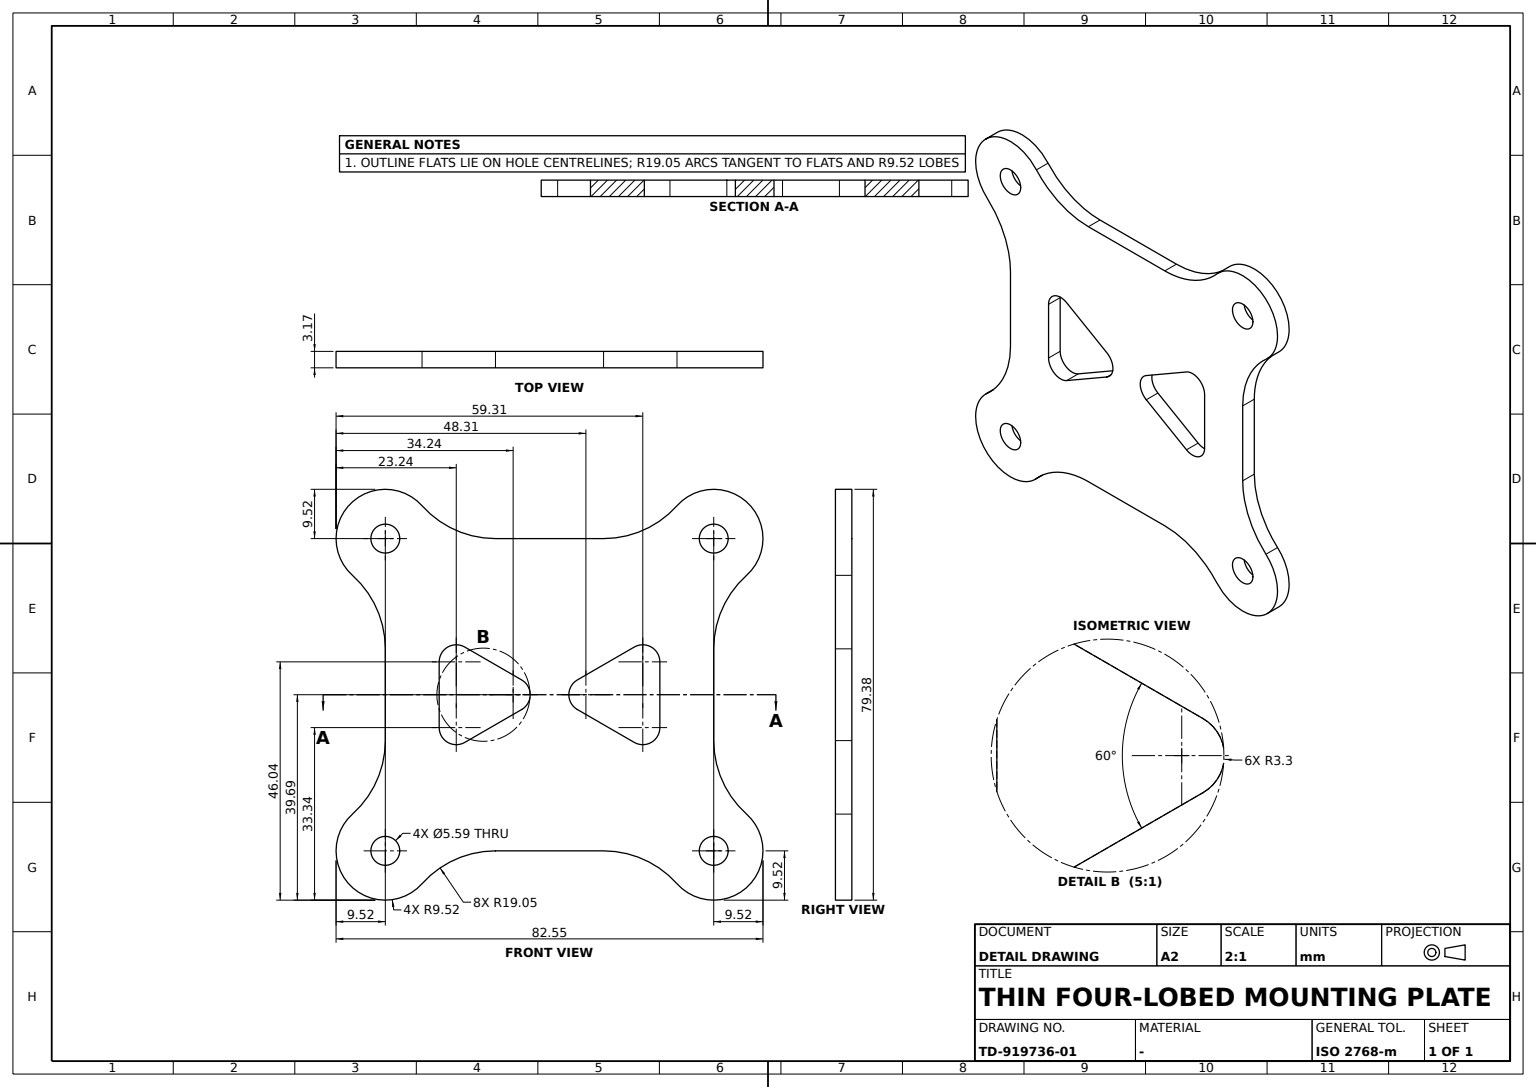
ISO-10303-21;
HEADER;
FILE_DESCRIPTION((''),'2;1');
FILE_NAME('','',(''),(''),'','','');
FILE_SCHEMA(('AUTOMOTIVE_DESIGN'));
ENDSEC;
DATA;
#1=APPLICATION_CONTEXT('');
#2=PRODUCT_CONTEXT('',#1,'mechanical');
#3=PRODUCT('','','',(#2));
#4=PRODUCT_DEFINITION_FORMATION('','',#3);
#5=PRODUCT_DEFINITION_CONTEXT('',#1,'design');
#6=PRODUCT_DEFINITION('','',#4,#5);
#7=PRODUCT_DEFINITION_SHAPE('','',#6);
#8=(LENGTH_UNIT()NAMED_UNIT(*)SI_UNIT(.MILLI.,.METRE.));
#9=(NAMED_UNIT(*)PLANE_ANGLE_UNIT()SI_UNIT($,.RADIAN.));
#10=(NAMED_UNIT(*)SI_UNIT($,.STERADIAN.)SOLID_ANGLE_UNIT());
#11=UNCERTAINTY_MEASURE_WITH_UNIT(LENGTH_MEASURE(1.E-05),#8,'distance_accuracy_value','');
#12=(GEOMETRIC_REPRESENTATION_CONTEXT(3)GLOBAL_UNCERTAINTY_ASSIGNED_CONTEXT((#11))GLOBAL_UNIT_ASSIGNED_CONTEXT((#8,#9,#10))REPRESENTATION_CONTEXT('',''));
#13=CARTESIAN_POINT('',(1.5875,34.544,-30.1625));
#14=VERTEX_POINT('',#13);
#15=CARTESIAN_POINT('',(1.5875,28.956,-30.1625));
#16=VERTEX_POINT('',#15);
#17=CARTESIAN_POINT('',(1.5875,31.75,-30.1625));
#18=DIRECTION('',(1.,0.,0.));
#19=DIRECTION('',(0.,1.,0.));
#20=AXIS2_PLACEMENT_3D('',#17,#18,#19);
#21=CIRCLE('',#20,2.794);
#22=EDGE_CURVE('',#14,#16,#21,.T.);
#23=ORIENTED_EDGE('',*,*,#22,.T.);
#24=CARTESIAN_POINT('',(-1.5875,28.956,-30.1625));
#25=VERTEX_POINT('',#24);
#26=CARTESIAN_POINT('',(-0.66,28.956,-30.1625));
#27=DIRECTION('',(-1.,0.,0.));
#28=VECTOR('',#27,1000.);
#29=LINE('',#26,#28);
#30=EDGE_CURVE('',#16,#25,#29,.T.);
#31=ORIENTED_EDGE('',*,*,#30,.T.);
#32=CARTESIAN_POINT('',(-1.5875,34.544,-30.1625));
#33=VERTEX_POINT('',#32);
#34=CARTESIAN_POINT('',(-1.5875,31.75,-30.1625));
#35=AXIS2_PLACEMENT_3D('',#34,#18,#19);
#36=CIRCLE('',#35,2.794);
#37=EDGE_CURVE('',#33,#25,#36,.T.);
#38=ORIENTED_EDGE('',*,*,#37,.F.);
#39=CARTESIAN_POINT('',(-0.66,34.544,-30.1625));
#40=LINE('',#39,#28);
#41=EDGE_CURVE('',#14,#33,#40,.T.);
#42=ORIENTED_EDGE('',*,*,#41,.F.);
#43=EDGE_LOOP('',(#23,#31,#38,#42));
#44=FACE_OUTER_BOUND('',#43,.T.);
#45=CARTESIAN_POINT('',(-0.66,31.75,-30.1625));
#46=AXIS2_PLACEMENT_3D('',#45,#27,#19);
#47=CYLINDRICAL_SURFACE('',#46,2.794);
#48=ADVANCED_FACE('',(#44),#47,.F.);
#49=CARTESIAN_POINT('',(1.5875,41.275,-30.1625));
#50=VERTEX_POINT('',#49);
#51=CARTESIAN_POINT('',(-1.5875,41.275,-30.1625));
#52=VERTEX_POINT('',#51);
#53=CARTESIAN_POINT('',(0.,41.275,-30.1625));
#54=LINE('',#53,#28);
#55=EDGE_CURVE('',#50,#52,#54,.T.);
#56=ORIENTED_EDGE('',*,*,#55,.F.);
#57=CARTESIAN_POINT('',(1.5875,24.650484,-36.5125));
#58=VERTEX_POINT('',#57);
#59=CIRCLE('',#20,9.525);
#60=EDGE_CURVE('',#58,#50,#59,.T.);
#61=ORIENTED_EDGE('',*,*,#60,.F.);
#62=CARTESIAN_POINT('',(-1.5875,24.650484,-36.5125));
#63=VERTEX_POINT('',#62);
#64=CARTESIAN_POINT('',(0.,24.650484,-36.5125));
#65=VECTOR('',#18,1000.);
#66=LINE('',#64,#65);
#67=EDGE_CURVE('',#63,#58,#66,.T.);
#68=ORIENTED_EDGE('',*,*,#67,.F.);
#69=CIRCLE('',#35,9.525);
#70=EDGE_CURVE('',#63,#52,#69,.T.);
#71=ORIENTED_EDGE('',*,*,#70,.T.);
#72=EDGE_LOOP('',(#56,#61,#68,#71));
#73=FACE_OUTER_BOUND('',#72,.T.);
#74=CARTESIAN_POINT('',(0.,31.75,-30.1625));
#75=AXIS2_PLACEMENT_3D('',#74,#27,#19);
#76=CYLINDRICAL_SURFACE('',#75,9.525);
#77=ADVANCED_FACE('',(#73),#76,.T.);
#78=CARTESIAN_POINT('',(1.5875,-31.75,8.863953));
#79=VERTEX_POINT('',#78);
#80=CARTESIAN_POINT('',(1.5875,-31.75,-8.863953));
#81=VERTEX_POINT('',#80);
#82=CARTESIAN_POINT('',(1.5875,-31.75,0.));
#83=DIRECTION('',(0.,0.,-1.));
#84=VECTOR('',#83,1000.);
#85=LINE('',#82,#84);
#86=EDGE_CURVE('',#79,#81,#85,.T.);
#87=ORIENTED_EDGE('',*,*,#86,.F.);
#88=CARTESIAN_POINT('',(-1.5875,-31.75,8.863953));
#89=VERTEX_POINT('',#88);
#90=CARTESIAN_POINT('',(0.,-31.75,8.863953));
#91=LINE('',#90,#28);
#92=EDGE_CURVE('',#79,#89,#91,.T.);
#93=ORIENTED_EDGE('',*,*,#92,.T.);
#94=CARTESIAN_POINT('',(-1.5875,-31.75,-8.863953));
#95=VERTEX_POINT('',#94);
#96=CARTESIAN_POINT('',(-1.5875,-31.75,0.));
#97=LINE('',#96,#84);
#98=EDGE_CURVE('',#89,#95,#97,.T.);
#99=ORIENTED_EDGE('',*,*,#98,.T.);
#100=CARTESIAN_POINT('',(0.,-31.75,-8.863953));
#101=LINE('',#100,#28);
#102=EDGE_CURVE('',#81,#95,#101,.T.);
#103=ORIENTED_EDGE('',*,*,#102,.F.);
#104=EDGE_LOOP('',(#87,#93,#99,#103));
#105=FACE_OUTER_BOUND('',#104,.T.);
#106=CARTESIAN_POINT('',(0.,-31.75,-30.1625));
#107=DIRECTION('',(0.,0.,1.));
#108=AXIS2_PLACEMENT_3D('',#106,#19,#107);
#109=PLANE('',#108);
#110=ADVANCED_FACE('',(#105),#109,.F.);
#111=ORIENTED_EDGE('',*,*,#67,.T.);
#112=CARTESIAN_POINT('',(1.5875,10.451453,-30.1625));
#113=VERTEX_POINT('',#112);
#114=CARTESIAN_POINT('',(1.5875,10.451453,-49.2125));
#115=AXIS2_PLACEMENT_3D('',#114,#27,#19);
#116=CIRCLE('',#115,19.05);
#117=EDGE_CURVE('',#113,#58,#116,.T.);
#118=ORIENTED_EDGE('',*,*,#117,.F.);
#119=CARTESIAN_POINT('',(-1.5875,10.451453,-30.1625));
#120=VERTEX_POINT('',#119);
#121=CARTESIAN_POINT('',(0.,10.451453,-30.1625));
#122=LINE('',#121,#65);
#123=EDGE_CURVE('',#120,#113,#122,.T.);
#124=ORIENTED_EDGE('',*,*,#123,.F.);
#125=CARTESIAN_POINT('',(-1.5875,10.451453,-49.2125));
#126=AXIS2_PLACEMENT_3D('',#125,#18,#19);
#127=CIRCLE('',#126,19.05);
#128=EDGE_CURVE('',#63,#120,#127,.T.);
#129=ORIENTED_EDGE('',*,*,#128,.F.);
#130=EDGE_LOOP('',(#111,#118,#124,#129));
#131=FACE_OUTER_BOUND('',#130,.T.);
#132=CARTESIAN_POINT('',(0.,10.451453,-49.2125));
#133=AXIS2_PLACEMENT_3D('',#132,#27,#107);
#134=CYLINDRICAL_SURFACE('',#133,19.05);
#135=ADVANCED_FACE('',(#131),#134,.F.);
#136=EDGE_CURVE('',#25,#33,#36,.T.);
#137=ORIENTED_EDGE('',*,*,#136,.F.);
#138=ORIENTED_EDGE('',*,*,#30,.F.);
#139=EDGE_CURVE('',#16,#14,#21,.T.);
#140=ORIENTED_EDGE('',*,*,#139,.T.);
#141=ORIENTED_EDGE('',*,*,#41,.T.);
#142=EDGE_LOOP('',(#137,#138,#140,#141));
#143=FACE_OUTER_BOUND('',#142,.T.);
#144=ADVANCED_FACE('',(#143),#47,.F.);
#145=CARTESIAN_POINT('',(1.5875,5.384477,-2.859616));
#146=VERTEX_POINT('',#145);
#147=CARTESIAN_POINT('',(-1.5875,5.384477,-2.859616));
#148=VERTEX_POINT('',#147);
#149=CARTESIAN_POINT('',(-0.66,5.384477,-2.859616));
#150=LINE('',#149,#28);
#151=EDGE_CURVE('',#146,#148,#150,.T.);
#152=ORIENTED_EDGE('',*,*,#151,.T.);
#153=CARTESIAN_POINT('',(-1.5875,5.384477,2.859616));
#154=VERTEX_POINT('',#153);
#155=CARTESIAN_POINT('',(-1.5875,7.035477,0.));
#156=AXIS2_PLACEMENT_3D('',#155,#18,#19);
#157=CIRCLE('',#156,3.302);
#158=EDGE_CURVE('',#154,#148,#157,.T.);
#159=ORIENTED_EDGE('',*,*,#158,.F.);
#160=CARTESIAN_POINT('',(1.5875,5.384477,2.859616));
#161=VERTEX_POINT('',#160);
#162=CARTESIAN_POINT('',(0.,5.384477,2.859616));
#163=LINE('',#162,#28);
#164=EDGE_CURVE('',#161,#154,#163,.T.);
#165=ORIENTED_EDGE('',*,*,#164,.F.);
#166=CARTESIAN_POINT('',(1.5875,7.035477,0.));
#167=AXIS2_PLACEMENT_3D('',#166,#18,#19);
#168=CIRCLE('',#167,3.302);
#169=EDGE_CURVE('',#161,#146,#168,.T.);
#170=ORIENTED_EDGE('',*,*,#169,.T.);
#171=EDGE_LOOP('',(#152,#159,#165,#170));
#172=FACE_OUTER_BOUND('',#171,.T.);
#173=CARTESIAN_POINT('',(-0.66,7.035477,0.));
#174=AXIS2_PLACEMENT_3D('',#173,#27,#19);
#175=CYLINDRICAL_SURFACE('',#174,3.302);
#176=ADVANCED_FACE('',(#172),#175,.F.);
#177=ORIENTED_EDGE('',*,*,#55,.T.);
#178=CARTESIAN_POINT('',(-1.5875,38.1,-23.062984));
#179=VERTEX_POINT('',#178);
#180=EDGE_CURVE('',#52,#179,#69,.T.);
#181=ORIENTED_EDGE('',*,*,#180,.T.);
#182=CARTESIAN_POINT('',(1.5875,38.1,-23.062984));
#183=VERTEX_POINT('',#182);
#184=CARTESIAN_POINT('',(0.,38.1,-23.062984));
#185=LINE('',#184,#28);
#186=EDGE_CURVE('',#183,#179,#185,.T.);
#187=ORIENTED_EDGE('',*,*,#186,.F.);
#188=EDGE_CURVE('',#50,#183,#59,.T.);
#189=ORIENTED_EDGE('',*,*,#188,.F.);
#190=EDGE_LOOP('',(#177,#181,#187,#189));
#191=FACE_OUTER_BOUND('',#190,.T.);
#192=ADVANCED_FACE('',(#191),#76,.T.);
#193=CARTESIAN_POINT('',(-1.5875,-10.451453,30.1625));
#194=VERTEX_POINT('',#193);
#195=CARTESIAN_POINT('',(1.5875,-10.451453,30.1625));
#196=VERTEX_POINT('',#195);
#197=CARTESIAN_POINT('',(0.,-10.451453,30.1625));
#198=LINE('',#197,#65);
#199=EDGE_CURVE('',#194,#196,#198,.T.);
#200=ORIENTED_EDGE('',*,*,#199,.F.);
#201=CARTESIAN_POINT('',(-1.5875,-24.650484,36.5125));
#202=VERTEX_POINT('',#201);
#203=CARTESIAN_POINT('',(-1.5875,-10.451453,49.2125));
#204=AXIS2_PLACEMENT_3D('',#203,#18,#19);
#205=CIRCLE('',#204,19.05);
#206=EDGE_CURVE('',#202,#194,#205,.T.);
#207=ORIENTED_EDGE('',*,*,#206,.F.);
#208=CARTESIAN_POINT('',(1.5875,-24.650484,36.5125));
#209=VERTEX_POINT('',#208);
#210=CARTESIAN_POINT('',(0.,-24.650484,36.5125));
#211=LINE('',#210,#65);
#212=EDGE_CURVE('',#202,#209,#211,.T.);
#213=ORIENTED_EDGE('',*,*,#212,.T.);
#214=CARTESIAN_POINT('',(1.5875,-10.451453,49.2125));
#215=AXIS2_PLACEMENT_3D('',#214,#27,#19);
#216=CIRCLE('',#215,19.05);
#217=EDGE_CURVE('',#196,#209,#216,.T.);
#218=ORIENTED_EDGE('',*,*,#217,.F.);
#219=EDGE_LOOP('',(#200,#207,#213,#218));
#220=FACE_OUTER_BOUND('',#219,.T.);
#221=CARTESIAN_POINT('',(0.,-10.451453,49.2125));
#222=AXIS2_PLACEMENT_3D('',#221,#27,#83);
#223=CYLINDRICAL_SURFACE('',#222,19.05);
#224=ADVANCED_FACE('',(#220),#223,.F.);
#225=CARTESIAN_POINT('',(1.5875,-38.1,-23.062984));
#226=VERTEX_POINT('',#225);
#227=CARTESIAN_POINT('',(1.5875,-41.275,-30.1625));
#228=VERTEX_POINT('',#227);
#229=CARTESIAN_POINT('',(1.5875,-31.75,-30.1625));
#230=AXIS2_PLACEMENT_3D('',#229,#18,#19);
#231=CIRCLE('',#230,9.525);
#232=EDGE_CURVE('',#226,#228,#231,.T.);
#233=ORIENTED_EDGE('',*,*,#232,.F.);
#234=CARTESIAN_POINT('',(-1.5875,-38.1,-23.062984));
#235=VERTEX_POINT('',#234);
#236=CARTESIAN_POINT('',(0.,-38.1,-23.062984));
#237=LINE('',#236,#28);
#238=EDGE_CURVE('',#226,#235,#237,.T.);
#239=ORIENTED_EDGE('',*,*,#238,.T.);
#240=CARTESIAN_POINT('',(-1.5875,-41.275,-30.1625));
#241=VERTEX_POINT('',#240);
#242=CARTESIAN_POINT('',(-1.5875,-31.75,-30.1625));
#243=AXIS2_PLACEMENT_3D('',#242,#18,#19);
#244=CIRCLE('',#243,9.525);
#245=EDGE_CURVE('',#235,#241,#244,.T.);
#246=ORIENTED_EDGE('',*,*,#245,.T.);
#247=CARTESIAN_POINT('',(0.,-41.275,-30.1625));
#248=LINE('',#247,#28);
#249=EDGE_CURVE('',#228,#241,#248,.T.);
#250=ORIENTED_EDGE('',*,*,#249,.F.);
#251=EDGE_LOOP('',(#233,#239,#246,#250));
#252=FACE_OUTER_BOUND('',#251,.T.);
#253=AXIS2_PLACEMENT_3D('',#106,#27,#19);
#254=CYLINDRICAL_SURFACE('',#253,9.525);
#255=ADVANCED_FACE('',(#252),#254,.T.);
#256=CARTESIAN_POINT('',(-1.5875,38.1,23.062984));
#257=VERTEX_POINT('',#256);
#258=CARTESIAN_POINT('',(-1.5875,31.75,8.863953));
#259=VERTEX_POINT('',#258);
#260=CARTESIAN_POINT('',(-1.5875,50.8,8.863953));
#261=AXIS2_PLACEMENT_3D('',#260,#18,#19);
#262=CIRCLE('',#261,19.05);
#263=EDGE_CURVE('',#257,#259,#262,.T.);
#264=ORIENTED_EDGE('',*,*,#263,.F.);
#265=CARTESIAN_POINT('',(1.5875,38.1,23.062984));
#266=VERTEX_POINT('',#265);
#267=CARTESIAN_POINT('',(0.,38.1,23.062984));
#268=LINE('',#267,#28);
#269=EDGE_CURVE('',#266,#257,#268,.T.);
#270=ORIENTED_EDGE('',*,*,#269,.F.);
#271=CARTESIAN_POINT('',(1.5875,31.75,8.863953));
#272=VERTEX_POINT('',#271);
#273=CARTESIAN_POINT('',(1.5875,50.8,8.863953));
#274=AXIS2_PLACEMENT_3D('',#273,#27,#19);
#275=CIRCLE('',#274,19.05);
#276=EDGE_CURVE('',#272,#266,#275,.T.);
#277=ORIENTED_EDGE('',*,*,#276,.F.);
#278=CARTESIAN_POINT('',(0.,31.75,8.863953));
#279=LINE('',#278,#28);
#280=EDGE_CURVE('',#272,#259,#279,.T.);
#281=ORIENTED_EDGE('',*,*,#280,.T.);
#282=EDGE_LOOP('',(#264,#270,#277,#281));
#283=FACE_OUTER_BOUND('',#282,.T.);
#284=CARTESIAN_POINT('',(0.,50.8,8.863953));
#285=DIRECTION('',(0.,-0.666666667,0.745355992));
#286=AXIS2_PLACEMENT_3D('',#284,#18,#285);
#287=CYLINDRICAL_SURFACE('',#286,19.05);
#288=ADVANCED_FACE('',(#283),#287,.F.);
#289=ORIENTED_EDGE('',*,*,#238,.F.);
#290=CARTESIAN_POINT('',(1.5875,-50.8,-8.863953));
#291=AXIS2_PLACEMENT_3D('',#290,#27,#19);
#292=CIRCLE('',#291,19.05);
#293=EDGE_CURVE('',#81,#226,#292,.T.);
#294=ORIENTED_EDGE('',*,*,#293,.F.);
#295=ORIENTED_EDGE('',*,*,#102,.T.);
#296=CARTESIAN_POINT('',(-1.5875,-50.8,-8.863953));
#297=AXIS2_PLACEMENT_3D('',#296,#18,#19);
#298=CIRCLE('',#297,19.05);
#299=EDGE_CURVE('',#235,#95,#298,.T.);
#300=ORIENTED_EDGE('',*,*,#299,.F.);
#301=EDGE_LOOP('',(#289,#294,#295,#300));
#302=FACE_OUTER_BOUND('',#301,.T.);
#303=CARTESIAN_POINT('',(0.,-50.8,-8.863953));
#304=DIRECTION('',(0.,0.666666667,-0.745355992));
#305=AXIS2_PLACEMENT_3D('',#303,#18,#304);
#306=CYLINDRICAL_SURFACE('',#305,19.05);
#307=ADVANCED_FACE('',(#302),#306,.F.);
#308=CARTESIAN_POINT('',(1.5875,-28.956,-30.1625));
#309=VERTEX_POINT('',#308);
#310=CARTESIAN_POINT('',(-1.5875,-28.956,-30.1625));
#311=VERTEX_POINT('',#310);
#312=CARTESIAN_POINT('',(-0.66,-28.956,-30.1625));
#313=LINE('',#312,#28);
#314=EDGE_CURVE('',#309,#311,#313,.T.);
#315=ORIENTED_EDGE('',*,*,#314,.F.);
#316=CARTESIAN_POINT('',(1.5875,-34.544,-30.1625));
#317=VERTEX_POINT('',#316);
#318=CIRCLE('',#230,2.794);
#319=EDGE_CURVE('',#309,#317,#318,.T.);
#320=ORIENTED_EDGE('',*,*,#319,.T.);
#321=CARTESIAN_POINT('',(-1.5875,-34.544,-30.1625));
#322=VERTEX_POINT('',#321);
#323=CARTESIAN_POINT('',(-0.66,-34.544,-30.1625));
#324=LINE('',#323,#28);
#325=EDGE_CURVE('',#317,#322,#324,.T.);
#326=ORIENTED_EDGE('',*,*,#325,.T.);
#327=CIRCLE('',#243,2.794);
#328=EDGE_CURVE('',#311,#322,#327,.T.);
#329=ORIENTED_EDGE('',*,*,#328,.F.);
#330=EDGE_LOOP('',(#315,#320,#326,#329));
#331=FACE_OUTER_BOUND('',#330,.T.);
#332=CARTESIAN_POINT('',(-0.66,-31.75,-30.1625));
#333=AXIS2_PLACEMENT_3D('',#332,#27,#19);
#334=CYLINDRICAL_SURFACE('',#333,2.794);
#335=ADVANCED_FACE('',(#331),#334,.F.);
#336=CARTESIAN_POINT('',(1.5875,-41.275,30.1625));
#337=VERTEX_POINT('',#336);
#338=CARTESIAN_POINT('',(1.5875,-31.75,30.1625));
#339=AXIS2_PLACEMENT_3D('',#338,#18,#19);
#340=CIRCLE('',#339,9.525);
#341=EDGE_CURVE('',#209,#337,#340,.T.);
#342=ORIENTED_EDGE('',*,*,#341,.F.);
#343=ORIENTED_EDGE('',*,*,#212,.F.);
#344=CARTESIAN_POINT('',(-1.5875,-41.275,30.1625));
#345=VERTEX_POINT('',#344);
#346=CARTESIAN_POINT('',(-1.5875,-31.75,30.1625));
#347=AXIS2_PLACEMENT_3D('',#346,#18,#19);
#348=CIRCLE('',#347,9.525);
#349=EDGE_CURVE('',#202,#345,#348,.T.);
#350=ORIENTED_EDGE('',*,*,#349,.T.);
#351=CARTESIAN_POINT('',(0.,-41.275,30.1625));
#352=LINE('',#351,#28);
#353=EDGE_CURVE('',#337,#345,#352,.T.);
#354=ORIENTED_EDGE('',*,*,#353,.F.);
#355=EDGE_LOOP('',(#342,#343,#350,#354));
#356=FACE_OUTER_BOUND('',#355,.T.);
#357=CARTESIAN_POINT('',(0.,-31.75,30.1625));
#358=AXIS2_PLACEMENT_3D('',#357,#27,#19);
#359=CYLINDRICAL_SURFACE('',#358,9.525);
#360=ADVANCED_FACE('',(#356),#359,.T.);
#361=CARTESIAN_POINT('',(1.5875,21.336,-6.35));
#362=VERTEX_POINT('',#361);
#363=CARTESIAN_POINT('',(-1.5875,21.336,-6.35));
#364=VERTEX_POINT('',#363);
#365=CARTESIAN_POINT('',(0.,21.336,-6.35));
#366=LINE('',#365,#28);
#367=EDGE_CURVE('',#362,#364,#366,.T.);
#368=ORIENTED_EDGE('',*,*,#367,.F.);
#369=CARTESIAN_POINT('',(1.5875,21.336,6.35));
#370=VERTEX_POINT('',#369);
#371=CARTESIAN_POINT('',(1.5875,21.336,0.));
#372=VECTOR('',#107,1000.);
#373=LINE('',#371,#372);
#374=EDGE_CURVE('',#362,#370,#373,.T.);
#375=ORIENTED_EDGE('',*,*,#374,.T.);
#376=CARTESIAN_POINT('',(-1.5875,21.336,6.35));
#377=VERTEX_POINT('',#376);
#378=CARTESIAN_POINT('',(0.,21.336,6.35));
#379=LINE('',#378,#28);
#380=EDGE_CURVE('',#370,#377,#379,.T.);
#381=ORIENTED_EDGE('',*,*,#380,.T.);
#382=CARTESIAN_POINT('',(-1.5875,21.336,0.));
#383=LINE('',#382,#372);
#384=EDGE_CURVE('',#364,#377,#383,.T.);
#385=ORIENTED_EDGE('',*,*,#384,.F.);
#386=EDGE_LOOP('',(#368,#375,#381,#385));
#387=FACE_OUTER_BOUND('',#386,.T.);
#388=DIRECTION('',(0.,-1.,0.));
#389=AXIS2_PLACEMENT_3D('',#361,#388,#107);
#390=PLANE('',#389);
#391=ADVANCED_FACE('',(#387),#390,.T.);
#392=CARTESIAN_POINT('',(-1.5875,-24.650484,-36.5125));
#393=VERTEX_POINT('',#392);
#394=EDGE_CURVE('',#241,#393,#244,.T.);
#395=ORIENTED_EDGE('',*,*,#394,.T.);
#396=CARTESIAN_POINT('',(1.5875,-24.650484,-36.5125));
#397=VERTEX_POINT('',#396);
#398=CARTESIAN_POINT('',(0.,-24.650484,-36.5125));
#399=LINE('',#398,#65);
#400=EDGE_CURVE('',#393,#397,#399,.T.);
#401=ORIENTED_EDGE('',*,*,#400,.T.);
#402=EDGE_CURVE('',#228,#397,#231,.T.);
#403=ORIENTED_EDGE('',*,*,#402,.F.);
#404=ORIENTED_EDGE('',*,*,#249,.T.);
#405=EDGE_LOOP('',(#395,#401,#403,#404));
#406=FACE_OUTER_BOUND('',#405,.T.);
#407=ADVANCED_FACE('',(#406),#254,.T.);
#408=CARTESIAN_POINT('',(1.5875,-28.956,30.1625));
#409=VERTEX_POINT('',#408);
#410=CARTESIAN_POINT('',(1.5875,-34.544,30.1625));
#411=VERTEX_POINT('',#410);
#412=CIRCLE('',#339,2.794);
#413=EDGE_CURVE('',#409,#411,#412,.T.);
#414=ORIENTED_EDGE('',*,*,#413,.T.);
#415=CARTESIAN_POINT('',(-1.5875,-34.544,30.1625));
#416=VERTEX_POINT('',#415);
#417=CARTESIAN_POINT('',(-0.66,-34.544,30.1625));
#418=LINE('',#417,#28);
#419=EDGE_CURVE('',#411,#416,#418,.T.);
#420=ORIENTED_EDGE('',*,*,#419,.T.);
#421=CARTESIAN_POINT('',(-1.5875,-28.956,30.1625));
#422=VERTEX_POINT('',#421);
#423=CIRCLE('',#347,2.794);
#424=EDGE_CURVE('',#422,#416,#423,.T.);
#425=ORIENTED_EDGE('',*,*,#424,.F.);
#426=CARTESIAN_POINT('',(-0.66,-28.956,30.1625));
#427=LINE('',#426,#28);
#428=EDGE_CURVE('',#409,#422,#427,.T.);
#429=ORIENTED_EDGE('',*,*,#428,.F.);
#430=EDGE_LOOP('',(#414,#420,#425,#429));
#431=FACE_OUTER_BOUND('',#430,.T.);
#432=CARTESIAN_POINT('',(-0.66,-31.75,30.1625));
#433=AXIS2_PLACEMENT_3D('',#432,#27,#19);
#434=CYLINDRICAL_SURFACE('',#433,2.794);
#435=ADVANCED_FACE('',(#431),#434,.F.);
#436=CARTESIAN_POINT('',(1.5875,31.75,-8.863953));
#437=VERTEX_POINT('',#436);
#438=CARTESIAN_POINT('',(1.5875,50.8,-8.863953));
#439=AXIS2_PLACEMENT_3D('',#438,#27,#19);
#440=CIRCLE('',#439,19.05);
#441=EDGE_CURVE('',#183,#437,#440,.T.);
#442=ORIENTED_EDGE('',*,*,#441,.F.);
#443=ORIENTED_EDGE('',*,*,#186,.T.);
#444=CARTESIAN_POINT('',(-1.5875,31.75,-8.863953));
#445=VERTEX_POINT('',#444);
#446=CARTESIAN_POINT('',(-1.5875,50.8,-8.863953));
#447=AXIS2_PLACEMENT_3D('',#446,#18,#19);
#448=CIRCLE('',#447,19.05);
#449=EDGE_CURVE('',#445,#179,#448,.T.);
#450=ORIENTED_EDGE('',*,*,#449,.F.);
#451=CARTESIAN_POINT('',(0.,31.75,-8.863953));
#452=LINE('',#451,#28);
#453=EDGE_CURVE('',#437,#445,#452,.T.);
#454=ORIENTED_EDGE('',*,*,#453,.F.);
#455=EDGE_LOOP('',(#442,#443,#450,#454));
#456=FACE_OUTER_BOUND('',#455,.T.);
#457=CARTESIAN_POINT('',(0.,50.8,-8.863953));
#458=AXIS2_PLACEMENT_3D('',#457,#18,#388);
#459=CYLINDRICAL_SURFACE('',#458,19.05);
#460=ADVANCED_FACE('',(#456),#459,.F.);
#461=CARTESIAN_POINT('',(-1.5875,-38.1,23.062984));
#462=VERTEX_POINT('',#461);
#463=CARTESIAN_POINT('',(-1.5875,-50.8,8.863953));
#464=AXIS2_PLACEMENT_3D('',#463,#18,#19);
#465=CIRCLE('',#464,19.05);
#466=EDGE_CURVE('',#89,#462,#465,.T.);
#467=ORIENTED_EDGE('',*,*,#466,.F.);
#468=ORIENTED_EDGE('',*,*,#92,.F.);
#469=CARTESIAN_POINT('',(1.5875,-38.1,23.062984));
#470=VERTEX_POINT('',#469);
#471=CARTESIAN_POINT('',(1.5875,-50.8,8.863953));
#472=AXIS2_PLACEMENT_3D('',#471,#27,#19);
#473=CIRCLE('',#472,19.05);
#474=EDGE_CURVE('',#470,#79,#473,.T.);
#475=ORIENTED_EDGE('',*,*,#474,.F.);
#476=CARTESIAN_POINT('',(0.,-38.1,23.062984));
#477=LINE('',#476,#28);
#478=EDGE_CURVE('',#470,#462,#477,.T.);
#479=ORIENTED_EDGE('',*,*,#478,.T.);
#480=EDGE_LOOP('',(#467,#468,#475,#479));
#481=FACE_OUTER_BOUND('',#480,.T.);
#482=CARTESIAN_POINT('',(0.,-50.8,8.863953));
#483=AXIS2_PLACEMENT_3D('',#482,#18,#19);
#484=CYLINDRICAL_SURFACE('',#483,19.05);
#485=ADVANCED_FACE('',(#481),#484,.F.);
#486=ORIENTED_EDGE('',*,*,#453,.T.);
#487=CARTESIAN_POINT('',(-1.5875,31.75,0.));
#488=LINE('',#487,#372);
#489=EDGE_CURVE('',#445,#259,#488,.T.);
#490=ORIENTED_EDGE('',*,*,#489,.T.);
#491=ORIENTED_EDGE('',*,*,#280,.F.);
#492=CARTESIAN_POINT('',(1.5875,31.75,0.));
#493=LINE('',#492,#372);
#494=EDGE_CURVE('',#437,#272,#493,.T.);
#495=ORIENTED_EDGE('',*,*,#494,.F.);
#496=EDGE_LOOP('',(#486,#490,#491,#495));
#497=FACE_OUTER_BOUND('',#496,.T.);
#498=CARTESIAN_POINT('',(0.,31.75,30.1625));
#499=AXIS2_PLACEMENT_3D('',#498,#388,#83);
#500=PLANE('',#499);
#501=ADVANCED_FACE('',(#497),#500,.F.);
#502=CARTESIAN_POINT('',(1.5875,24.650484,36.5125));
#503=VERTEX_POINT('',#502);
#504=CARTESIAN_POINT('',(1.5875,10.451453,30.1625));
#505=VERTEX_POINT('',#504);
#506=CARTESIAN_POINT('',(1.5875,10.451453,49.2125));
#507=AXIS2_PLACEMENT_3D('',#506,#27,#19);
#508=CIRCLE('',#507,19.05);
#509=EDGE_CURVE('',#503,#505,#508,.T.);
#510=ORIENTED_EDGE('',*,*,#509,.F.);
#511=CARTESIAN_POINT('',(-1.5875,24.650484,36.5125));
#512=VERTEX_POINT('',#511);
#513=CARTESIAN_POINT('',(0.,24.650484,36.5125));
#514=LINE('',#513,#65);
#515=EDGE_CURVE('',#512,#503,#514,.T.);
#516=ORIENTED_EDGE('',*,*,#515,.F.);
#517=CARTESIAN_POINT('',(-1.5875,10.451453,30.1625));
#518=VERTEX_POINT('',#517);
#519=CARTESIAN_POINT('',(-1.5875,10.451453,49.2125));
#520=AXIS2_PLACEMENT_3D('',#519,#18,#19);
#521=CIRCLE('',#520,19.05);
#522=EDGE_CURVE('',#518,#512,#521,.T.);
#523=ORIENTED_EDGE('',*,*,#522,.F.);
#524=CARTESIAN_POINT('',(0.,10.451453,30.1625));
#525=LINE('',#524,#65);
#526=EDGE_CURVE('',#518,#505,#525,.T.);
#527=ORIENTED_EDGE('',*,*,#526,.T.);
#528=EDGE_LOOP('',(#510,#516,#523,#527));
#529=FACE_OUTER_BOUND('',#528,.T.);
#530=CARTESIAN_POINT('',(0.,10.451453,49.2125));
#531=DIRECTION('',(0.,0.745355992,-0.666666667));
#532=AXIS2_PLACEMENT_3D('',#530,#27,#531);
#533=CYLINDRICAL_SURFACE('',#532,19.05);
#534=ADVANCED_FACE('',(#529),#533,.F.);
#535=ORIENTED_EDGE('',*,*,#263,.T.);
#536=ORIENTED_EDGE('',*,*,#489,.F.);
#537=ORIENTED_EDGE('',*,*,#449,.T.);
#538=ORIENTED_EDGE('',*,*,#180,.F.);
#539=ORIENTED_EDGE('',*,*,#70,.F.);
#540=ORIENTED_EDGE('',*,*,#128,.T.);
#541=CARTESIAN_POINT('',(-1.5875,-10.451453,-30.1625));
#542=VERTEX_POINT('',#541);
#543=CARTESIAN_POINT('',(-1.5875,0.,-30.1625));
#544=VECTOR('',#19,1000.);
#545=LINE('',#543,#544);
#546=EDGE_CURVE('',#542,#120,#545,.T.);
#547=ORIENTED_EDGE('',*,*,#546,.F.);
#548=CARTESIAN_POINT('',(-1.5875,-10.451453,-49.2125));
#549=AXIS2_PLACEMENT_3D('',#548,#18,#19);
#550=CIRCLE('',#549,19.05);
#551=EDGE_CURVE('',#542,#393,#550,.T.);
#552=ORIENTED_EDGE('',*,*,#551,.T.);
#553=ORIENTED_EDGE('',*,*,#394,.F.);
#554=ORIENTED_EDGE('',*,*,#245,.F.);
#555=ORIENTED_EDGE('',*,*,#299,.T.);
#556=ORIENTED_EDGE('',*,*,#98,.F.);
#557=ORIENTED_EDGE('',*,*,#466,.T.);
#558=EDGE_CURVE('',#345,#462,#348,.T.);
#559=ORIENTED_EDGE('',*,*,#558,.F.);
#560=ORIENTED_EDGE('',*,*,#349,.F.);
#561=ORIENTED_EDGE('',*,*,#206,.T.);
#562=CARTESIAN_POINT('',(-1.5875,0.,30.1625));
#563=VECTOR('',#388,1000.);
#564=LINE('',#562,#563);
#565=EDGE_CURVE('',#518,#194,#564,.T.);
#566=ORIENTED_EDGE('',*,*,#565,.F.);
#567=ORIENTED_EDGE('',*,*,#522,.T.);
#568=CARTESIAN_POINT('',(-1.5875,41.275,30.1625));
#569=VERTEX_POINT('',#568);
#570=CARTESIAN_POINT('',(-1.5875,31.75,30.1625));
#571=AXIS2_PLACEMENT_3D('',#570,#18,#19);
#572=CIRCLE('',#571,9.525);
#573=EDGE_CURVE('',#569,#512,#572,.T.);
#574=ORIENTED_EDGE('',*,*,#573,.F.);
#575=EDGE_CURVE('',#257,#569,#572,.T.);
#576=ORIENTED_EDGE('',*,*,#575,.F.);
#577=EDGE_LOOP('',(#535,#536,#537,#538,#539,#540,#547,#552,#553,#554,#555,#556,#557,#559,#560,#561,#566,#567,#574,#576));
#578=FACE_OUTER_BOUND('',#577,.T.);
#579=CARTESIAN_POINT('',(-1.5875,28.956,30.1625));
#580=VERTEX_POINT('',#579);
#581=CARTESIAN_POINT('',(-1.5875,34.544,30.1625));
#582=VERTEX_POINT('',#581);
#583=CIRCLE('',#571,2.794);
#584=EDGE_CURVE('',#580,#582,#583,.T.);
#585=ORIENTED_EDGE('',*,*,#584,.T.);
#586=EDGE_CURVE('',#582,#580,#583,.T.);
#587=ORIENTED_EDGE('',*,*,#586,.T.);
#588=EDGE_LOOP('',(#585,#587));
#589=FACE_BOUND('',#588,.T.);
#590=EDGE_CURVE('',#322,#311,#327,.T.);
#591=ORIENTED_EDGE('',*,*,#590,.T.);
#592=ORIENTED_EDGE('',*,*,#328,.T.);
#593=EDGE_LOOP('',(#591,#592));
#594=FACE_BOUND('',#593,.T.);
#595=CARTESIAN_POINT('',(-1.5875,-16.383,9.209616));
#596=VERTEX_POINT('',#595);
#597=CARTESIAN_POINT('',(-1.5875,-21.336,6.35));
#598=VERTEX_POINT('',#597);
#599=CARTESIAN_POINT('',(-1.5875,-18.034,6.35));
#600=AXIS2_PLACEMENT_3D('',#599,#18,#19);
#601=CIRCLE('',#600,3.302);
#602=EDGE_CURVE('',#596,#598,#601,.T.);
#603=ORIENTED_EDGE('',*,*,#602,.T.);
#604=CARTESIAN_POINT('',(-1.5875,-21.336,-6.35));
#605=VERTEX_POINT('',#604);
#606=CARTESIAN_POINT('',(-1.5875,-21.336,0.));
#607=LINE('',#606,#372);
#608=EDGE_CURVE('',#605,#598,#607,.T.);
#609=ORIENTED_EDGE('',*,*,#608,.F.);
#610=CARTESIAN_POINT('',(-1.5875,-16.383,-9.209616));
#611=VERTEX_POINT('',#610);
#612=CARTESIAN_POINT('',(-1.5875,-18.034,-6.35));
#613=AXIS2_PLACEMENT_3D('',#612,#18,#19);
#614=CIRCLE('',#613,3.302);
#615=EDGE_CURVE('',#605,#611,#614,.T.);
#616=ORIENTED_EDGE('',*,*,#615,.T.);
#617=CARTESIAN_POINT('',(-1.5875,-5.384477,-2.859616));
#618=VERTEX_POINT('',#617);
#619=CARTESIAN_POINT('',(-1.5875,-10.883739,-6.034616));
#620=DIRECTION('',(0.,0.866025404,0.5));
#621=VECTOR('',#620,1000.);
#622=LINE('',#619,#621);
#623=EDGE_CURVE('',#611,#618,#622,.T.);
#624=ORIENTED_EDGE('',*,*,#623,.T.);
#625=CARTESIAN_POINT('',(-1.5875,-3.733477,0.));
#626=VERTEX_POINT('',#625);
#627=CARTESIAN_POINT('',(-1.5875,-7.035477,0.));
#628=AXIS2_PLACEMENT_3D('',#627,#18,#19);
#629=CIRCLE('',#628,3.302);
#630=EDGE_CURVE('',#618,#626,#629,.T.);
#631=ORIENTED_EDGE('',*,*,#630,.T.);
#632=CARTESIAN_POINT('',(-1.5875,-5.384477,2.859616));
#633=VERTEX_POINT('',#632);
#634=EDGE_CURVE('',#626,#633,#629,.T.);
#635=ORIENTED_EDGE('',*,*,#634,.T.);
#636=CARTESIAN_POINT('',(-1.5875,-10.883739,6.034616));
#637=DIRECTION('',(0.,0.866025404,-0.5));
#638=VECTOR('',#637,1000.);
#639=LINE('',#636,#638);
#640=EDGE_CURVE('',#596,#633,#639,.T.);
#641=ORIENTED_EDGE('',*,*,#640,.F.);
#642=EDGE_LOOP('',(#603,#609,#616,#624,#631,#635,#641));
#643=FACE_BOUND('',#642,.T.);
#644=EDGE_CURVE('',#416,#422,#423,.T.);
#645=ORIENTED_EDGE('',*,*,#644,.T.);
#646=ORIENTED_EDGE('',*,*,#424,.T.);
#647=EDGE_LOOP('',(#645,#646));
#648=FACE_BOUND('',#647,.T.);
#649=CARTESIAN_POINT('',(-1.5875,16.383,-9.209616));
#650=VERTEX_POINT('',#649);
#651=CARTESIAN_POINT('',(-1.5875,18.034,-6.35));
#652=AXIS2_PLACEMENT_3D('',#651,#18,#19);
#653=CIRCLE('',#652,3.302);
#654=EDGE_CURVE('',#650,#364,#653,.T.);
#655=ORIENTED_EDGE('',*,*,#654,.T.);
#656=ORIENTED_EDGE('',*,*,#384,.T.);
#657=CARTESIAN_POINT('',(-1.5875,16.383,9.209616));
#658=VERTEX_POINT('',#657);
#659=CARTESIAN_POINT('',(-1.5875,18.034,6.35));
#660=AXIS2_PLACEMENT_3D('',#659,#18,#19);
#661=CIRCLE('',#660,3.302);
#662=EDGE_CURVE('',#377,#658,#661,.T.);
#663=ORIENTED_EDGE('',*,*,#662,.T.);
#664=CARTESIAN_POINT('',(-1.5875,10.883739,6.034616));
#665=DIRECTION('',(0.,-0.866025404,-0.5));
#666=VECTOR('',#665,1000.);
#667=LINE('',#664,#666);
#668=EDGE_CURVE('',#658,#154,#667,.T.);
#669=ORIENTED_EDGE('',*,*,#668,.T.);
#670=ORIENTED_EDGE('',*,*,#158,.T.);
#671=CARTESIAN_POINT('',(-1.5875,10.883739,-6.034616));
#672=LINE('',#671,#638);
#673=EDGE_CURVE('',#148,#650,#672,.T.);
#674=ORIENTED_EDGE('',*,*,#673,.T.);
#675=EDGE_LOOP('',(#655,#656,#663,#669,#670,#674));
#676=FACE_BOUND('',#675,.T.);
#677=ORIENTED_EDGE('',*,*,#37,.T.);
#678=ORIENTED_EDGE('',*,*,#136,.T.);
#679=EDGE_LOOP('',(#677,#678));
#680=FACE_BOUND('',#679,.T.);
#681=CARTESIAN_POINT('',(-1.5875,0.,0.));
#682=AXIS2_PLACEMENT_3D('',#681,#18,#19);
#683=PLANE('',#682);
#684=ADVANCED_FACE('',(#578,#589,#594,#643,#648,#676,#680),#683,.F.);
#685=CARTESIAN_POINT('',(1.5875,41.275,30.1625));
#686=VERTEX_POINT('',#685);
#687=CARTESIAN_POINT('',(1.5875,31.75,30.1625));
#688=AXIS2_PLACEMENT_3D('',#687,#18,#19);
#689=CIRCLE('',#688,9.525);
#690=EDGE_CURVE('',#266,#686,#689,.T.);
#691=ORIENTED_EDGE('',*,*,#690,.F.);
#692=ORIENTED_EDGE('',*,*,#269,.T.);
#693=ORIENTED_EDGE('',*,*,#575,.T.);
#694=CARTESIAN_POINT('',(0.,41.275,30.1625));
#695=LINE('',#694,#28);
#696=EDGE_CURVE('',#686,#569,#695,.T.);
#697=ORIENTED_EDGE('',*,*,#696,.F.);
#698=EDGE_LOOP('',(#691,#692,#693,#697));
#699=FACE_OUTER_BOUND('',#698,.T.);
#700=AXIS2_PLACEMENT_3D('',#498,#27,#19);
#701=CYLINDRICAL_SURFACE('',#700,9.525);
#702=ADVANCED_FACE('',(#699),#701,.T.);
#703=ORIENTED_EDGE('',*,*,#615,.F.);
#704=CARTESIAN_POINT('',(1.5875,-21.336,-6.35));
#705=VERTEX_POINT('',#704);
#706=CARTESIAN_POINT('',(-0.66,-21.336,-6.35));
#707=LINE('',#706,#28);
#708=EDGE_CURVE('',#705,#605,#707,.T.);
#709=ORIENTED_EDGE('',*,*,#708,.F.);
#710=CARTESIAN_POINT('',(1.5875,-16.383,-9.209616));
#711=VERTEX_POINT('',#710);
#712=CARTESIAN_POINT('',(1.5875,-18.034,-6.35));
#713=AXIS2_PLACEMENT_3D('',#712,#18,#19);
#714=CIRCLE('',#713,3.302);
#715=EDGE_CURVE('',#705,#711,#714,.T.);
#716=ORIENTED_EDGE('',*,*,#715,.T.);
#717=CARTESIAN_POINT('',(-0.66,-16.383,-9.209616));
#718=LINE('',#717,#28);
#719=EDGE_CURVE('',#711,#611,#718,.T.);
#720=ORIENTED_EDGE('',*,*,#719,.T.);
#721=EDGE_LOOP('',(#703,#709,#716,#720));
#722=FACE_OUTER_BOUND('',#721,.T.);
#723=CARTESIAN_POINT('',(-0.66,-18.034,-6.35));
#724=AXIS2_PLACEMENT_3D('',#723,#27,#19);
#725=CYLINDRICAL_SURFACE('',#724,3.302);
#726=ADVANCED_FACE('',(#722),#725,.F.);
#727=ORIENTED_EDGE('',*,*,#696,.T.);
#728=ORIENTED_EDGE('',*,*,#573,.T.);
#729=ORIENTED_EDGE('',*,*,#515,.T.);
#730=EDGE_CURVE('',#686,#503,#689,.T.);
#731=ORIENTED_EDGE('',*,*,#730,.F.);
#732=EDGE_LOOP('',(#727,#728,#729,#731));
#733=FACE_OUTER_BOUND('',#732,.T.);
#734=ADVANCED_FACE('',(#733),#701,.T.);
#735=ORIENTED_EDGE('',*,*,#565,.T.);
#736=ORIENTED_EDGE('',*,*,#199,.T.);
#737=CARTESIAN_POINT('',(1.5875,0.,30.1625));
#738=LINE('',#737,#563);
#739=EDGE_CURVE('',#505,#196,#738,.T.);
#740=ORIENTED_EDGE('',*,*,#739,.F.);
#741=ORIENTED_EDGE('',*,*,#526,.F.);
#742=EDGE_LOOP('',(#735,#736,#740,#741));
#743=FACE_OUTER_BOUND('',#742,.T.);
#744=AXIS2_PLACEMENT_3D('',#357,#83,#19);
#745=PLANE('',#744);
#746=ADVANCED_FACE('',(#743),#745,.F.);
#747=CARTESIAN_POINT('',(1.5875,-16.383,9.209616));
#748=VERTEX_POINT('',#747);
#749=CARTESIAN_POINT('',(0.,-16.383,9.209616));
#750=LINE('',#749,#28);
#751=EDGE_CURVE('',#748,#596,#750,.T.);
#752=ORIENTED_EDGE('',*,*,#751,.T.);
#753=ORIENTED_EDGE('',*,*,#640,.T.);
#754=CARTESIAN_POINT('',(1.5875,-5.384477,2.859616));
#755=VERTEX_POINT('',#754);
#756=CARTESIAN_POINT('',(-0.66,-5.384477,2.859616));
#757=LINE('',#756,#28);
#758=EDGE_CURVE('',#755,#633,#757,.T.);
#759=ORIENTED_EDGE('',*,*,#758,.F.);
#760=CARTESIAN_POINT('',(1.5875,-10.883739,6.034616));
#761=DIRECTION('',(0.,-0.866025404,0.5));
#762=VECTOR('',#761,1000.);
#763=LINE('',#760,#762);
#764=EDGE_CURVE('',#755,#748,#763,.T.);
#765=ORIENTED_EDGE('',*,*,#764,.T.);
#766=EDGE_LOOP('',(#752,#753,#759,#765));
#767=FACE_OUTER_BOUND('',#766,.T.);
#768=DIRECTION('',(0.,0.5,0.866025404));
#769=AXIS2_PLACEMENT_3D('',#747,#768,#637);
#770=PLANE('',#769);
#771=ADVANCED_FACE('',(#767),#770,.F.);
#772=ORIENTED_EDGE('',*,*,#22,.F.);
#773=ORIENTED_EDGE('',*,*,#139,.F.);
#774=EDGE_LOOP('',(#772,#773));
#775=FACE_BOUND('',#774,.T.);
#776=ORIENTED_EDGE('',*,*,#60,.T.);
#777=ORIENTED_EDGE('',*,*,#188,.T.);
#778=ORIENTED_EDGE('',*,*,#441,.T.);
#779=ORIENTED_EDGE('',*,*,#494,.T.);
#780=ORIENTED_EDGE('',*,*,#276,.T.);
#781=ORIENTED_EDGE('',*,*,#690,.T.);
#782=ORIENTED_EDGE('',*,*,#730,.T.);
#783=ORIENTED_EDGE('',*,*,#509,.T.);
#784=ORIENTED_EDGE('',*,*,#739,.T.);
#785=ORIENTED_EDGE('',*,*,#217,.T.);
#786=ORIENTED_EDGE('',*,*,#341,.T.);
#787=EDGE_CURVE('',#337,#470,#340,.T.);
#788=ORIENTED_EDGE('',*,*,#787,.T.);
#789=ORIENTED_EDGE('',*,*,#474,.T.);
#790=ORIENTED_EDGE('',*,*,#86,.T.);
#791=ORIENTED_EDGE('',*,*,#293,.T.);
#792=ORIENTED_EDGE('',*,*,#232,.T.);
#793=ORIENTED_EDGE('',*,*,#402,.T.);
#794=CARTESIAN_POINT('',(1.5875,-10.451453,-30.1625));
#795=VERTEX_POINT('',#794);
#796=CARTESIAN_POINT('',(1.5875,-10.451453,-49.2125));
#797=AXIS2_PLACEMENT_3D('',#796,#27,#19);
#798=CIRCLE('',#797,19.05);
#799=EDGE_CURVE('',#397,#795,#798,.T.);
#800=ORIENTED_EDGE('',*,*,#799,.T.);
#801=CARTESIAN_POINT('',(1.5875,0.,-30.1625));
#802=LINE('',#801,#544);
#803=EDGE_CURVE('',#795,#113,#802,.T.);
#804=ORIENTED_EDGE('',*,*,#803,.T.);
#805=ORIENTED_EDGE('',*,*,#117,.T.);
#806=EDGE_LOOP('',(#776,#777,#778,#779,#780,#781,#782,#783,#784,#785,#786,#788,#789,#790,#791,#792,#793,#800,#804,#805));
#807=FACE_OUTER_BOUND('',#806,.T.);
#808=ORIENTED_EDGE('',*,*,#319,.F.);
#809=EDGE_CURVE('',#317,#309,#318,.T.);
#810=ORIENTED_EDGE('',*,*,#809,.F.);
#811=EDGE_LOOP('',(#808,#810));
#812=FACE_BOUND('',#811,.T.);
#813=CARTESIAN_POINT('',(1.5875,28.956,30.1625));
#814=VERTEX_POINT('',#813);
#815=CARTESIAN_POINT('',(1.5875,34.544,30.1625));
#816=VERTEX_POINT('',#815);
#817=CIRCLE('',#688,2.794);
#818=EDGE_CURVE('',#814,#816,#817,.T.);
#819=ORIENTED_EDGE('',*,*,#818,.F.);
#820=EDGE_CURVE('',#816,#814,#817,.T.);
#821=ORIENTED_EDGE('',*,*,#820,.F.);
#822=EDGE_LOOP('',(#819,#821));
#823=FACE_BOUND('',#822,.T.);
#824=ORIENTED_EDGE('',*,*,#169,.F.);
#825=CARTESIAN_POINT('',(1.5875,16.383,9.209616));
#826=VERTEX_POINT('',#825);
#827=CARTESIAN_POINT('',(1.5875,10.883739,6.034616));
#828=LINE('',#827,#666);
#829=EDGE_CURVE('',#826,#161,#828,.T.);
#830=ORIENTED_EDGE('',*,*,#829,.F.);
#831=CARTESIAN_POINT('',(1.5875,18.034,6.35));
#832=AXIS2_PLACEMENT_3D('',#831,#18,#19);
#833=CIRCLE('',#832,3.302);
#834=EDGE_CURVE('',#370,#826,#833,.T.);
#835=ORIENTED_EDGE('',*,*,#834,.F.);
#836=ORIENTED_EDGE('',*,*,#374,.F.);
#837=CARTESIAN_POINT('',(1.5875,16.383,-9.209616));
#838=VERTEX_POINT('',#837);
#839=CARTESIAN_POINT('',(1.5875,18.034,-6.35));
#840=AXIS2_PLACEMENT_3D('',#839,#18,#19);
#841=CIRCLE('',#840,3.302);
#842=EDGE_CURVE('',#838,#362,#841,.T.);
#843=ORIENTED_EDGE('',*,*,#842,.F.);
#844=CARTESIAN_POINT('',(1.5875,10.883739,-6.034616));
#845=LINE('',#844,#638);
#846=EDGE_CURVE('',#146,#838,#845,.T.);
#847=ORIENTED_EDGE('',*,*,#846,.F.);
#848=EDGE_LOOP('',(#824,#830,#835,#836,#843,#847));
#849=FACE_BOUND('',#848,.T.);
#850=CARTESIAN_POINT('',(1.5875,-21.336,6.35));
#851=VERTEX_POINT('',#850);
#852=CARTESIAN_POINT('',(1.5875,-18.034,6.35));
#853=AXIS2_PLACEMENT_3D('',#852,#18,#19);
#854=CIRCLE('',#853,3.302);
#855=EDGE_CURVE('',#748,#851,#854,.T.);
#856=ORIENTED_EDGE('',*,*,#855,.F.);
#857=ORIENTED_EDGE('',*,*,#764,.F.);
#858=CARTESIAN_POINT('',(1.5875,-3.733477,0.));
#859=VERTEX_POINT('',#858);
#860=CARTESIAN_POINT('',(1.5875,-7.035477,0.));
#861=AXIS2_PLACEMENT_3D('',#860,#18,#19);
#862=CIRCLE('',#861,3.302);
#863=EDGE_CURVE('',#859,#755,#862,.T.);
#864=ORIENTED_EDGE('',*,*,#863,.F.);
#865=CARTESIAN_POINT('',(1.5875,-5.384477,-2.859616));
#866=VERTEX_POINT('',#865);
#867=EDGE_CURVE('',#866,#859,#862,.T.);
#868=ORIENTED_EDGE('',*,*,#867,.F.);
#869=CARTESIAN_POINT('',(1.5875,-10.883739,-6.034616));
#870=LINE('',#869,#621);
#871=EDGE_CURVE('',#711,#866,#870,.T.);
#872=ORIENTED_EDGE('',*,*,#871,.F.);
#873=ORIENTED_EDGE('',*,*,#715,.F.);
#874=CARTESIAN_POINT('',(1.5875,-21.336,0.));
#875=LINE('',#874,#84);
#876=EDGE_CURVE('',#851,#705,#875,.T.);
#877=ORIENTED_EDGE('',*,*,#876,.F.);
#878=EDGE_LOOP('',(#856,#857,#864,#868,#872,#873,#877));
#879=FACE_BOUND('',#878,.T.);
#880=ORIENTED_EDGE('',*,*,#413,.F.);
#881=EDGE_CURVE('',#411,#409,#412,.T.);
#882=ORIENTED_EDGE('',*,*,#881,.F.);
#883=EDGE_LOOP('',(#880,#882));
#884=FACE_BOUND('',#883,.T.);
#885=CARTESIAN_POINT('',(1.5875,0.,0.));
#886=AXIS2_PLACEMENT_3D('',#885,#18,#19);
#887=PLANE('',#886);
#888=ADVANCED_FACE('',(#775,#807,#812,#823,#849,#879,#884),#887,.T.);
#889=ORIENTED_EDGE('',*,*,#881,.T.);
#890=ORIENTED_EDGE('',*,*,#428,.T.);
#891=ORIENTED_EDGE('',*,*,#644,.F.);
#892=ORIENTED_EDGE('',*,*,#419,.F.);
#893=EDGE_LOOP('',(#889,#890,#891,#892));
#894=FACE_OUTER_BOUND('',#893,.T.);
#895=ADVANCED_FACE('',(#894),#434,.F.);
#896=ORIENTED_EDGE('',*,*,#867,.T.);
#897=CARTESIAN_POINT('',(-0.66,-3.733477,0.));
#898=LINE('',#897,#28);
#899=EDGE_CURVE('',#859,#626,#898,.T.);
#900=ORIENTED_EDGE('',*,*,#899,.T.);
#901=ORIENTED_EDGE('',*,*,#630,.F.);
#902=CARTESIAN_POINT('',(0.,-5.384477,-2.859616));
#903=LINE('',#902,#28);
#904=EDGE_CURVE('',#866,#618,#903,.T.);
#905=ORIENTED_EDGE('',*,*,#904,.F.);
#906=EDGE_LOOP('',(#896,#900,#901,#905));
#907=FACE_OUTER_BOUND('',#906,.T.);
#908=CARTESIAN_POINT('',(-0.66,-7.035477,0.));
#909=AXIS2_PLACEMENT_3D('',#908,#27,#19);
#910=CYLINDRICAL_SURFACE('',#909,3.302);
#911=ADVANCED_FACE('',(#907),#910,.F.);
#912=ORIENTED_EDGE('',*,*,#123,.T.);
#913=ORIENTED_EDGE('',*,*,#803,.F.);
#914=CARTESIAN_POINT('',(0.,-10.451453,-30.1625));
#915=LINE('',#914,#65);
#916=EDGE_CURVE('',#542,#795,#915,.T.);
#917=ORIENTED_EDGE('',*,*,#916,.F.);
#918=ORIENTED_EDGE('',*,*,#546,.T.);
#919=EDGE_LOOP('',(#912,#913,#917,#918));
#920=FACE_OUTER_BOUND('',#919,.T.);
#921=AXIS2_PLACEMENT_3D('',#74,#107,#388);
#922=PLANE('',#921);
#923=ADVANCED_FACE('',(#920),#922,.F.);
#924=ORIENTED_EDGE('',*,*,#876,.T.);
#925=ORIENTED_EDGE('',*,*,#708,.T.);
#926=ORIENTED_EDGE('',*,*,#608,.T.);
#927=CARTESIAN_POINT('',(-0.66,-21.336,6.35));
#928=LINE('',#927,#28);
#929=EDGE_CURVE('',#851,#598,#928,.T.);
#930=ORIENTED_EDGE('',*,*,#929,.F.);
#931=EDGE_LOOP('',(#924,#925,#926,#930));
#932=FACE_OUTER_BOUND('',#931,.T.);
#933=AXIS2_PLACEMENT_3D('',#704,#388,#107);
#934=PLANE('',#933);
#935=ADVANCED_FACE('',(#932),#934,.F.);
#936=ORIENTED_EDGE('',*,*,#164,.T.);
#937=ORIENTED_EDGE('',*,*,#668,.F.);
#938=CARTESIAN_POINT('',(-0.66,16.383,9.209616));
#939=LINE('',#938,#28);
#940=EDGE_CURVE('',#826,#658,#939,.T.);
#941=ORIENTED_EDGE('',*,*,#940,.F.);
#942=ORIENTED_EDGE('',*,*,#829,.T.);
#943=EDGE_LOOP('',(#936,#937,#941,#942));
#944=FACE_OUTER_BOUND('',#943,.T.);
#945=DIRECTION('',(0.,0.5,-0.866025404));
#946=AXIS2_PLACEMENT_3D('',#825,#945,#665);
#947=PLANE('',#946);
#948=ADVANCED_FACE('',(#944),#947,.T.);
#949=CARTESIAN_POINT('',(0.,16.383,-9.209616));
#950=LINE('',#949,#28);
#951=EDGE_CURVE('',#838,#650,#950,.T.);
#952=ORIENTED_EDGE('',*,*,#951,.F.);
#953=ORIENTED_EDGE('',*,*,#842,.T.);
#954=ORIENTED_EDGE('',*,*,#367,.T.);
#955=ORIENTED_EDGE('',*,*,#654,.F.);
#956=EDGE_LOOP('',(#952,#953,#954,#955));
#957=FACE_OUTER_BOUND('',#956,.T.);
#958=CARTESIAN_POINT('',(-0.66,18.034,-6.35));
#959=AXIS2_PLACEMENT_3D('',#958,#27,#19);
#960=CYLINDRICAL_SURFACE('',#959,3.302);
#961=ADVANCED_FACE('',(#957),#960,.F.);
#962=CARTESIAN_POINT('',(-0.66,34.544,30.1625));
#963=LINE('',#962,#28);
#964=EDGE_CURVE('',#816,#582,#963,.T.);
#965=ORIENTED_EDGE('',*,*,#964,.T.);
#966=ORIENTED_EDGE('',*,*,#584,.F.);
#967=CARTESIAN_POINT('',(-0.66,28.956,30.1625));
#968=LINE('',#967,#28);
#969=EDGE_CURVE('',#814,#580,#968,.T.);
#970=ORIENTED_EDGE('',*,*,#969,.F.);
#971=ORIENTED_EDGE('',*,*,#818,.T.);
#972=EDGE_LOOP('',(#965,#966,#970,#971));
#973=FACE_OUTER_BOUND('',#972,.T.);
#974=CARTESIAN_POINT('',(-0.66,31.75,30.1625));
#975=AXIS2_PLACEMENT_3D('',#974,#27,#19);
#976=CYLINDRICAL_SURFACE('',#975,2.794);
#977=ADVANCED_FACE('',(#973),#976,.F.);
#978=ORIENTED_EDGE('',*,*,#904,.T.);
#979=ORIENTED_EDGE('',*,*,#623,.F.);
#980=ORIENTED_EDGE('',*,*,#719,.F.);
#981=ORIENTED_EDGE('',*,*,#871,.T.);
#982=EDGE_LOOP('',(#978,#979,#980,#981));
#983=FACE_OUTER_BOUND('',#982,.T.);
#984=DIRECTION('',(0.,-0.5,0.866025404));
#985=AXIS2_PLACEMENT_3D('',#710,#984,#620);
#986=PLANE('',#985);
#987=ADVANCED_FACE('',(#983),#986,.T.);
#988=ORIENTED_EDGE('',*,*,#602,.F.);
#989=ORIENTED_EDGE('',*,*,#751,.F.);
#990=ORIENTED_EDGE('',*,*,#855,.T.);
#991=ORIENTED_EDGE('',*,*,#929,.T.);
#992=EDGE_LOOP('',(#988,#989,#990,#991));
#993=FACE_OUTER_BOUND('',#992,.T.);
#994=CARTESIAN_POINT('',(-0.66,-18.034,6.35));
#995=AXIS2_PLACEMENT_3D('',#994,#27,#19);
#996=CYLINDRICAL_SURFACE('',#995,3.302);
#997=ADVANCED_FACE('',(#993),#996,.F.);
#998=ORIENTED_EDGE('',*,*,#758,.T.);
#999=ORIENTED_EDGE('',*,*,#634,.F.);
#1000=ORIENTED_EDGE('',*,*,#899,.F.);
#1001=ORIENTED_EDGE('',*,*,#863,.T.);
#1002=EDGE_LOOP('',(#998,#999,#1000,#1001));
#1003=FACE_OUTER_BOUND('',#1002,.T.);
#1004=ADVANCED_FACE('',(#1003),#910,.F.);
#1005=ORIENTED_EDGE('',*,*,#916,.T.);
#1006=ORIENTED_EDGE('',*,*,#799,.F.);
#1007=ORIENTED_EDGE('',*,*,#400,.F.);
#1008=ORIENTED_EDGE('',*,*,#551,.F.);
#1009=EDGE_LOOP('',(#1005,#1006,#1007,#1008));
#1010=FACE_OUTER_BOUND('',#1009,.T.);
#1011=CARTESIAN_POINT('',(0.,-10.451453,-49.2125));
#1012=DIRECTION('',(0.,-0.745355992,0.666666667));
#1013=AXIS2_PLACEMENT_3D('',#1011,#27,#1012);
#1014=CYLINDRICAL_SURFACE('',#1013,19.05);
#1015=ADVANCED_FACE('',(#1010),#1014,.F.);
#1016=ORIENTED_EDGE('',*,*,#380,.F.);
#1017=ORIENTED_EDGE('',*,*,#834,.T.);
#1018=ORIENTED_EDGE('',*,*,#940,.T.);
#1019=ORIENTED_EDGE('',*,*,#662,.F.);
#1020=EDGE_LOOP('',(#1016,#1017,#1018,#1019));
#1021=FACE_OUTER_BOUND('',#1020,.T.);
#1022=CARTESIAN_POINT('',(-0.66,18.034,6.35));
#1023=AXIS2_PLACEMENT_3D('',#1022,#27,#19);
#1024=CYLINDRICAL_SURFACE('',#1023,3.302);
#1025=ADVANCED_FACE('',(#1021),#1024,.F.);
#1026=ORIENTED_EDGE('',*,*,#353,.T.);
#1027=ORIENTED_EDGE('',*,*,#558,.T.);
#1028=ORIENTED_EDGE('',*,*,#478,.F.);
#1029=ORIENTED_EDGE('',*,*,#787,.F.);
#1030=EDGE_LOOP('',(#1026,#1027,#1028,#1029));
#1031=FACE_OUTER_BOUND('',#1030,.T.);
#1032=ADVANCED_FACE('',(#1031),#359,.T.);
#1033=ORIENTED_EDGE('',*,*,#846,.T.);
#1034=ORIENTED_EDGE('',*,*,#951,.T.);
#1035=ORIENTED_EDGE('',*,*,#673,.F.);
#1036=ORIENTED_EDGE('',*,*,#151,.F.);
#1037=EDGE_LOOP('',(#1033,#1034,#1035,#1036));
#1038=FACE_OUTER_BOUND('',#1037,.T.);
#1039=AXIS2_PLACEMENT_3D('',#145,#768,#637);
#1040=PLANE('',#1039);
#1041=ADVANCED_FACE('',(#1038),#1040,.T.);
#1042=ORIENTED_EDGE('',*,*,#969,.T.);
#1043=ORIENTED_EDGE('',*,*,#586,.F.);
#1044=ORIENTED_EDGE('',*,*,#964,.F.);
#1045=ORIENTED_EDGE('',*,*,#820,.T.);
#1046=EDGE_LOOP('',(#1042,#1043,#1044,#1045));
#1047=FACE_OUTER_BOUND('',#1046,.T.);
#1048=ADVANCED_FACE('',(#1047),#976,.F.);
#1049=ORIENTED_EDGE('',*,*,#809,.T.);
#1050=ORIENTED_EDGE('',*,*,#314,.T.);
#1051=ORIENTED_EDGE('',*,*,#590,.F.);
#1052=ORIENTED_EDGE('',*,*,#325,.F.);
#1053=EDGE_LOOP('',(#1049,#1050,#1051,#1052));
#1054=FACE_OUTER_BOUND('',#1053,.T.);
#1055=ADVANCED_FACE('',(#1054),#334,.F.);
#1056=CLOSED_SHELL('',(#48,#77,#110,#135,#144,#176,#192,#224,#255,#288,#307,#335,#360,#391,#407,#435,#460,#485,#501,#534,#684,#702,#726,#734,#746,#771,#888,#895,#911,#923,#935,#948,#961,#977,#987,#997,#1004,#1015,#1025,#1032,#1041,#1048,#1055));
#1057=MANIFOLD_SOLID_BREP('',#1056);
#1058=ADVANCED_BREP_SHAPE_REPRESENTATION('',(#1057),#12);
#1059=SHAPE_DEFINITION_REPRESENTATION(#7,#1058);
ENDSEC;
END-ISO-10303-21;
